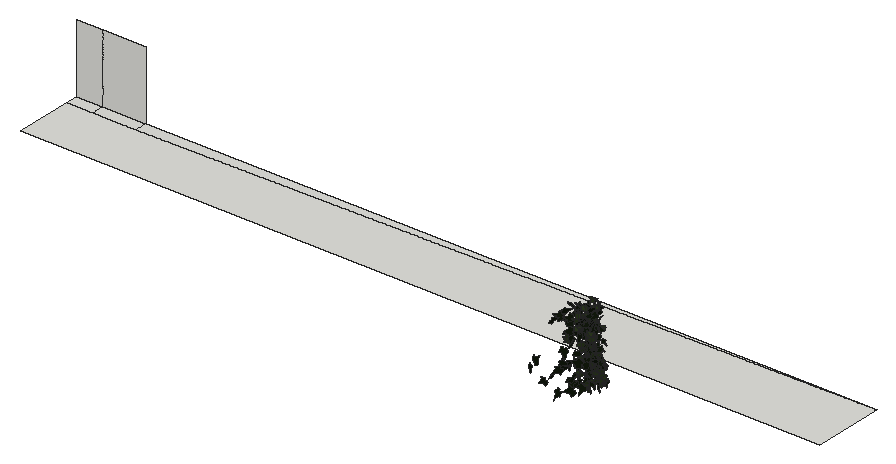
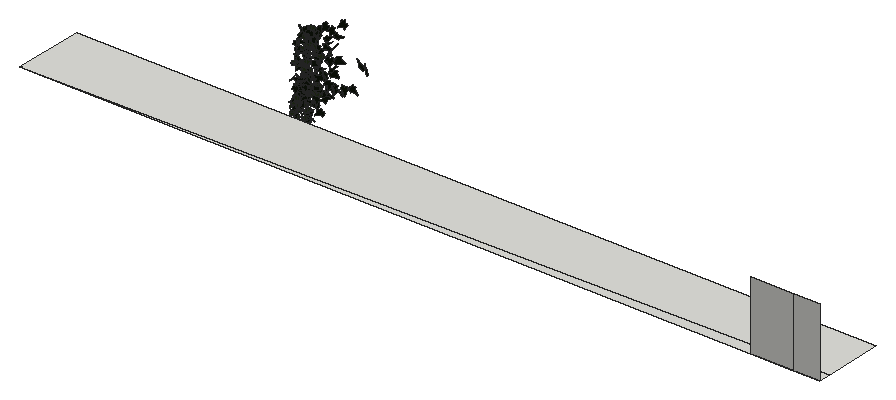
# SketchUp Ruby script. Lengths in inches.
U = 1.inch
M = Sketchup.active_model
def pt(a) = Geom::Point3d.new(a.map { |v| v * U })
def face(e, loops, mat)
  f = e.add_face(loops[0].map { |a| pt(a) })
  loops[1..].each { |l| e.add_face(l.map { |a| pt(a) }).erase! }
  f.material = f.back_material = mat if mat
  f
end
# faces: each face lists its corners as indices into pts; further lists are holes
def faces(e, pts, list, mat = nil) = list.each { |f| face(e, (f[0].is_a?(Array) ? f : [f]).map { |l| l.map { |i| pts[i] } }, mat) }
# xy, xz, yz: faces in a plane at the given z, y or x. An outline is a flat list of corners, or four numbers for a rectangle; further outlines are holes
def ring(l) = l.size == 4 ? [[l[0], l[1]], [l[2], l[1]], [l[2], l[3]], [l[0], l[3]]] : l.each_slice(2).to_a
def flat(e, list, mat, &to3) = list.each { |f| face(e, (f[0].is_a?(Array) ? f : [f]).map { |l| ring(l).map { |u, v| to3.(u, v) } }, mat) }
def xy(e, z, list, mat = nil) = flat(e, list, mat) { |x, y| [x, y, z] }
def xz(e, y, list, mat = nil) = flat(e, list, mat) { |x, z| [x, y, z] }
def yz(e, x, list, mat = nil) = flat(e, list, mat) { |y, z| [x, y, z] }
def lines(e, pts, list) = list.each { |a, b| e.add_line(pt(pts[a]), pt(pts[b])) }
# prism: a flat outline (further loops are holes) pulled along v
def prism(e, loops, v, mat = nil)
  f = face(e, loops, mat); d = Geom::Vector3d.new(v.map { |x| x * U })
  f.pushpull(f.normal.samedirection?(d) ? d.length : -d.length)
end
def box(e, o, s, mat = nil) = prism(e, [[o, [o[0] + s[0], o[1], o[2]], [o[0] + s[0], o[1] + s[1], o[2]], [o[0], o[1] + s[1], o[2]]]], [0, 0, s[2]], mat)
def at(x, y, z, deg = 0) = Geom::Transformation.translation(pt([x, y, z])) * Geom::Transformation.rotation(ORIGIN, Z_AXIS, deg.degrees)
def axes(o, x, y, z) = Geom::Transformation.new([*x, 0, *y, 0, *z, 0, *pt(o).to_a, 1])
def part(name) = M.definitions.add(name)
# library, detail: a bought-in or finely detailed component or shape, given as its bounding box
def library(name, o, s) = part(name).tap { |d| box(d.entities, o, s) }
def detail(e, o, s) = box(e.add_group.entities, o, s)
def put(e, d, t, mat = nil) = e.add_instance(d, t).tap { |i| i.material = mat if mat }
def group(e, t, mat = nil) = e.add_group.tap { |g| g.transformation = t; g.material = mat if mat }.entities
root = M.entities
M.materials.add("efeu1").color = [18, 25, 13]
M.materials.add("efeu2").color = [43, 57, 29]
c1 = part("ivyleaf_9")
p = [[1.54,2.16,1.25],[1.36,2.04,1.19],[-0.21,0.99,0.68],[-0.71,1.11,0.82],[-0.85,0.86,0.67],[-0.8,0.17,0.21],
  [-0.9,-0.01,0.1],[-0.67,-0.16,-0.02],[-0.08,-0.08,-0.05],[-0.03,-0.6,-0.4],[0.65,-0.88,-0.66],[0.83,-0.6,-0.49],
  [1.29,-0.42,-0.43],[1.8125,-0.07,-0.26],[1.21,0.44,0.15]]
faces(c1.entities,p,[[0,1,2,3,4,5,6,7,8,9,10,11,12,13,14]],"efeu1")
c2 = part("ivyleaf_10")
p = [[0,0.5,-0.03],[-0.0625,2.02,-0.43],[-0.19,2.01,-0.46],[-0.54,1.05,-0.29],[-0.52,0.625,-0.18],[-0.83,0.76,-0.28],
  [-1.16,0.64,-0.33],[-1.15,0.33,-0.24],[-0.77,-0.39,0.02],[-0.3,-0.51,0.16],[0.04,-0.48,0.23],[-0.02,2.01,-0.4375],
  [-0.06,2.01,-0.43],[0.04,-0.49,0.23],[0.67,-0.49,0.14],[1.38,0.36,-0.2],[1.375,0.51,-0.24],[0.81,0.65,-0.19],
  [0.62,0.59,-0.15],[0.6,1.09,-0.28],[0.5,1.23,-0.31]]
faces(c2.entities,p,[[0,1,2,3,4,5,6,7,8,9,10],[11,12,0,13,14,15,16,17,18,19,20]],"efeu2")
xy(root,212.04,[[222.91,139.625,222.91,166.9375,255.63,166.9375,600,172.6875,600,139.625],[222.91,166.9375,235.22,172.6875],[235.22,166.9375,255.63,172.6875],[255.63,166.9375,255.63,172.6875,600,172.6875]])
xz(root,172.6875,[[222.91,212.04,235.22,244.35],[235.22,212.04,255.63,244.35]])
put(root,c1,axes([489.04,107.25,219.34],[-0.10171,0.33302,1.23895],[0.37987,-1.13822,0.35983],[1.28078,0.36403,-0.00833]))
put(root,c1,axes([490.16,108.75,221.96],[-0.5052,0.59256,1.08878],[0.68053,-0.83616,0.78501],[1.10672,0.78465,0.01431]))
put(root,c1,axes([491.3,122.97,236.84],[0.60854,-1.02373,-0.20138],[-0.03753,0.20155,-1.21337],[1.12461,0.56068,0.06847]))
put(root,c1,axes([492.44,122.89,218.13],[0.00554,0.22522,1.15832],[-0.28561,1.08343,-0.22658],[-1.19352,-0.25822,0.0596]))
put(root,c1,axes([492.76,111.33,214.01],[0.17278,0.17118,-1.1899],[-1.04476,-0.61365,-0.23616],[-0.68521,0.97881,0.06004]))
put(root,c1,axes([493.82,114.29,214.9],[-0.08217,1.18063,0.10076],[-0.01963,0.09591,-1.23034],[-1.27922,-0.0773,0.01241]))
put(root,c1,axes([494.79,118.48,238.45],[-0.64696,-0.31659,-0.96088],[-0.78751,-0.5761,0.69698],[-0.70174,0.9384,0.10371]))
put(root,c1,axes([494.4,122.13,230.3],[0.37874,1.0301,-0.29598],[-0.09362,-0.27112,-1.13167],[-1.15038,0.3612,-0.00535]))
put(root,c1,axes([494.75,127.88,235.37],[-0.39311,-0.35611,0.92517],[-0.58208,-0.71072,-0.52523],[0.85566,-0.64709,0.06774]))
put(root,c1,axes([494.61,135.09,209.74],[-0.35512,-0.73439,0.18051],[-0.06081,-0.17104,-0.81552],[0.7538,-0.35977,0.01925]))
put(root,c1,axes([495.09,134.37,208.07],[-0.2856,0.78411,0.05143],[-0.00592,0.05257,-0.83441],[-0.78577,-0.28539,-0.0124]))
put(root,c2,axes([494.82,134.58,209.49],[-0.74125,-0.3012,-0.23294],[0.22767,0.05803,-0.79952],[0.30521,-0.77482,0.03067]))
put(root,c2,axes([495.11,126.38,233.46],[-1.07293,-0.21408,0.10536],[-0.11451,0.01138,-1.05635],[0.22873,-0.99855,-0.03462]))
put(root,c1,axes([495.25,134.47,212.06],[-0.74459,-0.40023,0.0405],[0.06147,-0.19741,-0.82066],[0.39755,-0.71908,0.20275]))
put(root,c1,axes([494.92,134.7,208.4],[-0.01052,-0.81612,-0.20319],[-0.01922,0.20338,-0.81591],[0.84081,-0.00556,-0.02119]))
put(root,c1,axes([494.39,118.89,216.28],[0.4027,0.73789,-0.93408],[0.35266,0.83876,0.85764],[1.20483,-0.49214,0.06117]))
put(root,c1,axes([495.07,123.52,223.59],[-0.43715,1.00274,0.10617],[0.02617,-0.1003,1.1245],[1.08825,0.40522,0.0156]))
put(root,c1,axes([495.72,128.53,216.39],[-0.01838,1.02527,0.09743],[-0.1177,0.09137,-1.06061],[-1.10566,-0.02677,0.11129]))
put(root,c2,axes([495.24,134.92,208.11],[0.52925,0.64171,-0.07514],[-0.05706,-0.05033,-0.83172],[-0.64357,0.53218,0.01194]))
put(root,c1,axes([495.95,133.42,216.8125],[-0.78489,-0.15812,0.33707],[-0.31655,-0.13059,-0.79838],[0.19599,-0.84417,0.06037]))
put(root,c2,axes([495.66,135,209.41],[0.3353,-0.66129,-0.38228],[-0.04268,0.40061,-0.73044],[0.76263,0.31316,0.1272]))
put(root,c2,axes([495.7,134.72,210.81],[0.07658,-0.84372,-0.04713],[0.00665,0.04792,-0.84712],[0.84501,0.07609,0.01093]))
put(root,c2,axes([495.69,133.97,213.78],[0.35332,0.70703,-0.3529],[-0.21969,-0.28344,-0.78782],[-0.75905,0.41114,0.06375]))
put(root,c2,axes([496.22,120.92,227.69],[0.43574,0.65548,0.79497],[-0.4783,-0.62404,0.79963],[0.97668,-0.59804,0.03693]))
put(root,c1,axes([495.8125,111.77,240.32],[-0.17706,0.50903,-1.10678],[-0.31093,1.02469,0.55585],[1.23554,0.33081,-0.01872]))
put(root,c1,axes([495.32,119.21,240.76],[0.36831,0.76242,-0.76182],[0.21461,0.70974,0.86447],[1.12152,-0.38619,0.08475]))
put(root,c1,axes([495.51,119.29,224.43],[0.02529,-1.31148,-0.08317],[0.02017,0.08031,-1.364],[1.41888,0.02224,0.02088]))
put(root,c1,axes([495.9,120.45,218.71],[1.00104,0.79642,-0.22113],[-0.17622,-0.13636,-1.27093],[-0.87265,0.94114,0.00298]))
put(root,c1,axes([496.11,134.12,218.96],[-0.67862,-0.51522,-0.21541],[0.17418,0.12681,-0.85204],[0.53058,-0.70061,0.00419]))
put(root,c1,axes([496.35,121.51,215.83],[-0.00738,-0.02583,1.12303],[0.13343,1.07275,0.0275],[-1.1589,0.12368,-0.00399]))
put(root,c2,axes([495.9,128.08,217.55],[0.55185,0.78022,0.48086],[0.16955,0.4466,-0.96419],[-0.9647,0.52481,0.10562]))
put(root,c1,axes([495.68,122.23,235.11],[-0.42552,-0.38668,-1.13477],[0.95435,0.6441,-0.56924],[0.80764,-0.96484,0.07477]))
put(root,c2,axes([496.41,134.01,216.16],[0.10607,-0.86802,0.02616],[0.03421,-0.02215,-0.87392],[0.86774,0.10697,0.03125]))
put(root,c1,axes([496.66,134,223.16],[0.03161,0.8889,-0.11605],[-0.0938,-0.11221,-0.885],[-0.89153,0.04333,0.08899]))
put(root,c1,axes([497.13,121.32,237.29],[-0.34227,-0.13974,1.01438],[-0.9724,-0.37511,-0.36014],[0.43225,-0.9545,-0.00698]))
put(root,c1,axes([496.23,134.41,219.35],[0.81492,0.33541,0.00747],[0.00913,-0.00256,-0.88122],[-0.33537,0.81495,-0.00584]))
put(root,c1,axes([496.87,132.89,222],[-0.8299,-0.28092,-0.1811],[0.16449,0.07871,-0.8759],[0.29096,-0.84578,-0.02136]))
put(root,c2,axes([496.56,127.25,240.54],[-0.52467,0.90112,-0.27806],[0.09577,-0.25568,-1.06379],[-1.01061,-0.49205,0.04355]))
put(root,c2,axes([496.87,119.94,230.12],[0.1837,0.49778,-1.0049],[-0.27761,-0.93184,-0.54632],[-1.14059,0.30697,-0.02888]))
put(root,c1,axes([496.47,134.1875,216.04],[0.82755,0.25066,0.12672],[0.11325,0.06301,-0.86426],[-0.25703,0.83482,0.02718]))
put(root,c1,axes([497.01,132.18,223.83],[0.6338,0.33055,-0.55532],[-0.56454,-0.09539,-0.7011],[-0.31455,0.83724,0.13936]))
put(root,c2,axes([496.85,133.9,222.86],[-0.28737,-0.74179,-0.41221],[0.19652,0.36521,-0.7942],[0.82556,-0.34514,0.04557]))
put(root,c1,axes([496.72,131.95,219.43],[-0.59525,-0.24803,-0.60884],[0.63437,-0.00111,-0.61976],[0.17257,-0.85148,0.17816]))
put(root,c1,axes([497.27,130.99,224.3125],[-0.70407,0.42179,-0.39466],[0.28516,-0.28731,-0.81579],[-0.50234,-0.75427,0.09004]))
put(root,c1,axes([496.58,121.4375,243.24],[1.26723,-0.02604,-0.14385],[-0.1492,0.00917,-1.22058],[0.02908,1.18145,0.0063]))
put(root,c1,axes([497.53,116.6,220.98],[0.0176,0.40263,-1.05478],[-0.18674,-1.00056,-0.41599],[-1.16362,0.16666,0.05081]))
put(root,c2,axes([497.49,133.57,222.47],[-0.28073,0.77431,0.37785],[-0.48797,0.18463,-0.7409],[-0.71008,-0.433,0.35977]))
put(root,c1,axes([497.18,134.35,212.86],[-0.38053,-0.65159,0.39941],[0.01313,-0.45169,-0.72437],[0.76415,-0.31672,0.21134]))
put(root,c2,axes([497.77,124.78,228.36],[-0.49792,0.36679,0.90054],[-0.69462,0.58056,-0.6119],[-0.74093,-0.79076,-0.03153]))
put(root,c1,axes([496.55,124.66,208.33],[-0.12706,-0.23054,-1.1665],[0.80548,0.84016,-0.26095],[0.93841,-0.75236,0.06604]))
put(root,c2,axes([497.17,130.19,222.05],[0.03241,0.77652,0.47703],[0.03444,0.47594,-0.7771],[-0.91069,0.04563,-0.01241]))
put(root,c1,axes([496.93,121.52,230.01],[0.03418,-1.08707,0.40155],[0.00759,-0.38606,-1.13102],[1.24587,0.03217,-0.00413]))
put(root,c2,axes([497.3,129.8125,227.94],[-0.66296,0.75601,-0.01249],[0.01752,-0.00229,-1.01273],[-0.8164,-0.61397,-0.0116]))
put(root,c1,axes([498.02,129.76,207.95],[-1.02692,0.09772,-0.02308],[0.01806,-0.05412,-0.99262],[-0.10671,-0.94957,0.0542]))
put(root,c1,axes([498.33,129.82,217.5625],[-0.68141,0.55611,0.37114],[-0.47007,0.02148,-0.83511],[-0.53694,-0.72455,0.26011]))
put(root,c1,axes([497.4,134.97,208.01],[0.12814,-0.82287,0.0192],[-0.01266,-0.0214,-0.83264],[0.82299,0.1278,-0.0158]))
put(root,c1,axes([497.09,124.03,229.93],[0.17337,0.05719,1.19004],[1.09141,0.53733,-0.17537],[-0.58299,1.02294,0.02558]))
put(root,c2,axes([498.13,129.73,217.26],[-0.66019,-0.61668,0.06954],[-0.04787,-0.05063,-0.90339],[0.61874,-0.66191,0.00431]))
put(root,c1,axes([498.33,124.97,240.39],[-0.17221,-0.17296,0.99814],[-0.73804,-0.67397,-0.2444],[0.75138,-0.70164,-0.0113]))
put(root,c2,axes([498.1,132.97,227.38],[0.4241,-0.81769,-0.1481],[0.01828,0.17541,-0.91614],[0.8308,0.41356,0.09576]))
put(root,c1,axes([497.87,120.74,211.82],[-0.44173,-1.07457,-0.32087],[0.08631,0.29958,-1.19534],[1.20434,-0.4156,-0.03202]))
put(root,c1,axes([497.61,129.2,209.98],[1.05315,0.04965,0.01164],[0.0104,0.03101,-1.01496],[-0.05398,0.97471,0.0317]))
put(root,c2,axes([498.61,126.66,236.45],[0.77714,-0.37747,-0.70181],[-0.62806,0.34334,-0.84463],[0.55036,0.92482,0.02712]))
put(root,c1,axes([498.61,132.15,234.54],[-0.94064,-0.1192,-0.01452],[0.0258,-0.08869,-0.94377],[0.11727,-0.93656,0.09122]))
put(root,c1,axes([499.03,130.09,234.77],[-0.73853,0.4433,0.41509],[-0.3527,0.21893,-0.86134],[-0.49439,-0.8184,-0.00558]))
put(root,c1,axes([497.59,123.98,242.3125],[1.19558,-0.32993,0.12373],[0.14956,0.04925,-1.19798],[0.34801,1.1123,0.08975]))
put(root,c2,axes([498.48,133.2,227.78],[0.14103,-0.68346,-0.59855],[0.015,0.60739,-0.69002],[0.90838,0.09608,0.10432]))
put(root,c1,axes([499.19,126.16,228.85],[-0.13747,-0.04116,-1.01678],[-0.77798,-0.66334,0.12658],[-0.71528,0.7294,0.05774]))
put(root,c1,axes([498.89,119.32,233.1],[-0.37167,-0.2722,1.10926],[-0.7985,-0.77075,-0.45266],[0.88076,-0.81363,0.05771]))
put(root,c1,axes([499.12,123.29,240.79],[-0.1657,0.99448,0.58892],[-0.33728,0.51327,-1.02545],[-1.18904,-0.28418,0.20881]))
put(root,c1,axes([498.4,129.68,217.16],[0.08554,-0.13683,-0.93531],[-0.31118,0.85248,-0.16128],[0.93187,0.29723,0.032]))
put(root,c1,axes([498.97,130.38,209.625],[-0.11439,-0.78391,-0.54757],[-0.0898,-0.52001,0.8226],[-1.0159,0.13424,-0.01106]))
put(root,c1,axes([498.09,123.8125,220.88],[-0.30373,-0.18235,1.16396],[1.16529,0.31165,0.33477],[-0.3767,1.1111,0.09712]))
put(root,c1,axes([498.4,129.6875,225.82],[-0.16275,-0.92079,0.03748],[-0.00431,-0.0373,-0.93506],[0.92155,-0.16279,0.00225]))
put(root,c1,axes([499.3,124.7,224.89],[-0.63767,0.25231,-0.72477],[-0.70711,0.24001,0.66728],[0.37513,0.88129,0.02578]))
put(root,c1,axes([499.5625,127.11,224.41],[-0.69135,0.61207,0.60328],[-0.48856,0.36537,-0.92012],[-0.7686,-0.78279,0.04223]))
put(root,c1,axes([499.15,111.75,211.05],[-1.31922,0.09386,-0.42953],[0.44102,-0.07361,-1.27343],[-0.1214,-1.28733,0.04149]))
put(root,c2,axes([498.31,123.35,232.8],[0.69691,0.48531,0.5784],[0.48562,0.32737,-0.83968],[-0.63219,0.78646,-0.00739]))
put(root,c1,axes([498.31,130.29,207.71],[0.98175,-0.29555,-0.03879],[-0.03963,0.00775,-0.9941],[0.31927,0.90976,-0.00413]))
put(root,c1,axes([498.77,123.82,234.75],[0.65604,0.73331,0.15794],[0.08164,0.13449,-0.9899],[-0.80464,0.61152,0.02833]))
put(root,c2,axes([498.38,132.61,229.54],[0.73165,0.15383,0.57334],[0.54485,0.1872,-0.74551],[-0.23564,0.91049,0.05641]))
put(root,c1,axes([498.29,132.42,225.6875],[0.81378,0.08466,0.41578],[0.41416,0.03703,-0.81815],[-0.09225,0.91309,-0.00537]))
put(root,c1,axes([497.98,122.87,216.52],[1.07921,-0.48847,0.50036],[0.46667,-0.21156,-1.15676],[0.57491,1.08869,-0.00029]))
put(root,c1,axes([499.36,123.89,224.65],[0.15653,-0.90706,0.60586],[-0.10099,0.57501,0.95531],[-1.15988,-0.17248,-0.00141]))
put(root,c2,axes([498.44,123.09,218.04],[-0.60621,0.16778,-0.87248],[0.8574,-0.27182,-0.60896],[-0.34438,-0.97209,0.01969]))
put(root,c1,axes([498.65,129.76,239.6],[-0.02126,0.17413,0.96713],[0.2079,-0.90994,0.18144],[1.00041,0.1928,-0.01716]))
put(root,c1,axes([499.57,124.65,217.37],[-0.85023,-0.42758,0.44075],[-0.397,-0.21111,-0.93166],[0.51491,-0.8688,0.00946]))
put(root,c2,axes([498.71,122.86,213.92],[0.25345,0.54074,0.79376],[0.31051,0.70709,-0.61294],[-0.9613,0.37097,0.01129]))
put(root,c1,axes([498.53,124.3,209.86],[-0.08457,0.11147,1.02734],[0.5133,-0.8661,0.14082],[0.94297,0.48146,0.01548]))
put(root,c1,axes([499.43,126.4375,234.16],[-0.91658,0.28737,-0.32972],[0.31554,-0.12533,-0.93154],[-0.33764,-0.89726,0.02452]))
put(root,c2,axes([498.6875,129.87,224.97],[-0.03678,0.0072,-0.99469],[0.77939,0.62828,-0.02181],[0.67793,-0.72193,-0.0289]))
put(root,c2,axes([499.7,130.89,242.03],[-0.86623,0.10035,0.44623],[-0.45699,-0.15074,-0.85322],[-0.01874,-0.96268,0.18012]))
put(root,c1,axes([498.98,131.43,235.375],[-0.37926,-0.79752,-0.36037],[0.43282,0.17043,-0.83269],[0.76064,-0.49463,0.29413]))
put(root,c2,axes([499.33,130.51,238.68],[-0.32152,0.82464,-0.3916],[-0.10297,-0.44529,-0.85315],[-0.90707,-0.24175,0.23566]))
put(root,c2,axes([499.96,131,215.89],[-0.06646,0.03335,0.96104],[-0.87996,0.43597,-0.07279],[-0.47222,-0.8171,0.00039]))
put(root,c1,axes([499.8,124.54,233.64],[-0.92479,0.61939,-0.34605],[0.27773,-0.21212,-1.09889],[-0.70674,-0.89384,0.02098]))
put(root,c1,axes([498.875,129.97,223.84],[0.50252,-0.83473,-0.05917],[-0.02961,0.04985,-0.99388],[0.90311,0.4661,0.00033]))
put(root,c1,axes([499.74,132.2,236.03],[-0.90783,-0.27021,-0.19313],[0.22187,-0.07509,-0.93788],[0.24716,-0.92511,0.13254]))
put(root,c2,axes([499.2,124.12,220.125],[-0.90232,-0.07225,-0.58232],[0.60577,0.00764,-0.87144],[0.06942,-1.00573,0.03521]))
put(root,c2,axes([499.66,125.43,223.32],[-0.07199,-0.9255,-0.07265],[0.01646,0.06894,-0.96495],[1.00225,-0.0676,0.01062]))
put(root,c2,axes([499.49,129.3,230.98],[0.70318,0.75871,0.0404],[0.02931,0.0279,-1.03977],[-0.81995,0.65166,-0.00252]))
put(root,c2,axes([499.82,134.2,214.39],[-0.0503,-0.85595,-0.12657],[0.01219,0.12607,-0.85742],[0.86517,-0.05154,0.00473]))
put(root,c2,axes([499.85,128.72,233.84],[0.71613,-0.71314,-0.30994],[-0.10482,0.31273,-1.00286],[0.82813,0.65628,0.14108]))
put(root,c2,axes([499.95,134.36,214.45],[-0.40499,-0.74938,0.15285],[-0.01894,-0.16308,-0.8497],[0.76457,-0.40098,0.05992]))
put(root,c1,axes([499.93,131.25,218.58],[0.34181,0.85227,0.09917],[0.05588,0.08248,-0.94528],[-0.92451,0.32008,-0.02047]))
put(root,c1,axes([499.32,123.07,239.6875],[1.02219,-0.59304,-0.23328],[-0.19368,0.13617,-1.16141],[0.6568,0.96311,0.02057]))
put(root,c1,axes([500.04,126.3,223.77],[0.39361,-0.25395,-0.97233],[-0.82974,0.53277,-0.46197],[0.63742,0.85033,-0.00094]))
put(root,c2,axes([499.13,130.65,206.77],[0.36879,-0.05761,-0.91913],[0.95424,-0.04302,0.35796],[-0.06582,-0.94648,0.03967]))
put(root,c2,axes([500.18,127.18,227.8],[-0.22906,0.76849,-0.55779],[-0.13167,0.5226,0.8289],[1.00351,0.24399,-0.01856]))
put(root,c2,axes([500,125.29,233.5625],[0.73235,-0.86183,-0.05062],[-0.03016,0.03995,-1.14048],[0.93177,0.67867,0.00287]))
put(root,c1,axes([500.54,128.22,234.75],[-1.10687,0.01128,0.1043],[-0.10892,-0.07671,-1.0629],[-0.00402,-1.02692,0.08054]))
put(root,c1,axes([500.25,124.22,240.49],[-0.84758,0.38507,-0.43315],[0.38508,-0.21808,-0.90842],[-0.47644,-0.86129,0.03636]))
put(root,c1,axes([499.29,129.29,226.3],[0.89534,-0.08112,0.40909],[0.42318,-0.03468,-0.86629],[0.09521,0.91695,0.00343]))
put(root,c2,axes([500,127.57,240.4],[0.79665,-0.58142,0.10459],[0.08195,-0.06513,-0.98625],[0.58504,0.80084,-0.00427]))
put(root,c2,axes([500.64,121.92,216.85],[0.29042,0.1278,-1.06263],[-0.61613,0.89763,-0.03938],[0.92582,0.55728,0.30712]))
put(root,c2,axes([500.31,127.6875,237.49],[0.90473,0.43672,-0.47132],[-0.46007,-0.16194,-0.98123],[-0.50035,0.93857,0.05]))
put(root,c1,axes([500.22,132.2,213.98],[-0.65736,-0.56371,0.30057],[0.00351,-0.40358,-0.81153],[0.68415,-0.53956,0.29297]))
put(root,c1,axes([499.77,134.38,213.53],[0.18804,-0.83335,0.10377],[0.02658,-0.10038,-0.85429],[0.83937,0.18987,0.0038]))
put(root,c2,axes([500.24,131.89,206.17],[0.34971,-0.768,-0.16209],[-0.04525,0.15743,-0.84355],[0.78362,0.35183,0.02362]))
put(root,c1,axes([499.79,127.06,230.91],[0.00482,-1.05742,-0.21449],[0.06454,0.20616,-1.09798],[1.16174,-0.00706,0.06189]))
put(root,c2,axes([500.48,134.13,217.45],[-0.83334,-0.16244,0.23055],[-0.22327,-0.05944,-0.84889],[0.17232,-0.8626,0.01508]))
put(root,c1,axes([500.22,126.62,241.625],[0.95183,0.51386,-0.41668],[-0.41265,-0.13836,-1.05864],[-0.57004,0.95818,0.0706]))
put(root,c1,axes([501.03,126.5625,218.49],[-0.11909,0.13228,1.03811],[-1.08526,0.04933,-0.12224],[-0.06908,-1.00304,0.13089]))
put(root,c1,axes([499.875,120.2,221.66],[1.02073,-0.44715,-0.33369],[-0.30803,0.14737,-1.08732],[0.50834,0.98716,0.01118]))
put(root,c1,axes([500.74,127.13,217.28],[-0.90946,-0.36324,0.22394],[0.21293,0.08658,0.95378],[-0.40329,0.86487,-0.00143]))
put(root,c1,axes([499.94,132.99,229.65],[0.11086,-0.7358,-0.55565],[0.19262,0.56579,-0.7108],[0.90169,-0.0304,0.22016]))
put(root,c2,axes([500.59,123.18,226.77],[-0.7352,-0.8394,-0.00642],[0.00081,0.00734,-1.12396],[0.90657,-0.68073,-0.0042]))
put(root,c1,axes([500.38,131.3,226.98],[-0.72438,0.01747,-0.59204],[0.60661,-0.12536,-0.69224],[-0.10187,-0.87076,0.08778]))
put(root,c1,axes([500.18,123.42,237.36],[0.96949,0.66828,0.08804],[0.06339,0.06291,-1.16377],[-0.72474,0.89946,0.01599]))
put(root,c2,axes([500.23,126.6,229.84],[-0.81521,0.49077,-0.41504],[0.33017,-0.2609,-0.93505],[-0.59807,-0.81299,0.04952]))
put(root,c2,axes([500.28,125.84,235.4],[0.1232,0.97799,0.3591],[0.05441,0.34174,-1.02395],[-1.1188,0.12431,-0.01025]))
put(root,c2,axes([500.61,126.45,240.15],[-1.0373,-0.50003,-0.02992],[0.03191,0.00553,-1.1261],[0.53998,-0.96088,0.00908]))
put(root,c1,axes([501.2,127.39,214.9],[-0.42348,-0.43714,-0.68184],[-0.47872,-0.48309,0.6107],[-0.70361,0.59178,-0.00513]))
put(root,c2,axes([500.46,122.3,219.9375],[-1.10661,0.21848,-0.1847],[0.19035,-0.02497,-1.0895],[-0.23713,-1.03961,-0.01265]))
put(root,c2,axes([501.0625,127.57,224.48],[-0.95947,-0.0351,0.55145],[-0.57126,-0.04074,-0.92448],[0.05509,-1.0338,0.01771]))
put(root,c1,axes([501.09,109.86,222.25],[-0.16495,0.06879,-1.34198],[-0.07788,-1.29778,-0.06308],[-1.3934,0.06439,0.16239]))
put(root,c1,axes([501.3,128.23,226.96],[-0.48672,0.61917,0.55677],[-0.33589,0.43577,-0.79644],[-0.81771,-0.54755,-0.00425]))
put(root,c2,axes([500.96,129.78,223.26],[0.1073,-0.04662,-0.96659],[-0.27998,0.89631,-0.07558],[0.96524,0.26516,0.08553]))
put(root,c2,axes([500.41,126.34,221.6],[-0.03099,-0.2925,-0.90066],[0.27162,-0.83553,0.28483],[-0.94911,-0.22956,0.11092]))
put(root,c1,axes([501.7,116.54,210.55],[-0.26535,-0.1554,-1.33294],[-0.8372,-1.02556,0.28387],[-1.11503,0.80701,0.10406]))
put(root,c1,axes([501.11,132.09,219.73],[-0.01644,0.19408,-0.85097],[-0.13778,-0.80944,-0.1972],[-0.89771,0.12068,0.04585]))
put(root,c2,axes([500.72,125.92,222.78],[-0.06477,0.74956,0.74363],[-0.10384,0.70911,-0.78147],[-1.11395,-0.10969,0.02961]))
put(root,c1,axes([500.48,126.78,218.94],[0.07833,0.4036,-0.82541],[0.05053,0.79347,0.42408],[0.9603,-0.07467,0.04502]))
put(root,c2,axes([500.72,126.43,224.0625],[-0.00898,0.31388,-0.87062],[0.00354,-0.83716,-0.32647],[-0.96556,-0.00599,0.0069]))
put(root,c1,axes([501.39,127.68,237.18],[-0.09006,-0.06986,-1.0053],[-0.33642,-0.9168,0.09686],[-0.99115,0.31753,0.05847]))
put(root,c1,axes([501.68,125.23,216.78],[-0.20404,0.03206,1.03357],[-1.07156,0.06039,-0.19818],[-0.07056,-1.00981,0.02097]))
put(root,c1,axes([500.52,132.64,231.51],[0.21833,-0.91678,-0.02062],[-0.00221,0.02067,-0.94241],[0.91701,0.21832,0.00263]))
put(root,c1,axes([501.29,125.91,236.4],[0.41034,-0.0779,-0.95814],[-0.98447,0.13505,-0.40284],[0.16703,0.98737,-0.02049]))
put(root,c2,axes([501.1,122.58,214.65],[-0.19101,-0.9346,0.42419],[-0.03944,-0.40789,-0.9885],[1.1006,-0.17682,0.03819]))
put(root,c1,axes([501.7,125.24,235.02],[-1.17464,0.07906,0.29967],[-0.31322,-0.01765,-1.13345],[-0.07763,-1.12501,0.03885]))
put(root,c1,axes([500.32,128.9,224.71],[0.67119,-0.73828,0.24572],[0.18848,-0.16179,-1.0032],[0.81568,0.64489,0.02962]))
put(root,c1,axes([501.53,131.75,216.58],[-0.6096,0.69623,0.10403],[-0.05269,0.0892,-0.93195],[-0.75782,-0.56626,-0.01889]))
put(root,c1,axes([500.98,126.9,224.11],[-0.5552,-0.89143,0.00533],[-0.00254,-0.00456,-1.0702],[0.96275,-0.51408,0.00025]))
put(root,c1,axes([501.39,132.51,233.31],[-0.12939,0.76527,0.37778],[-0.02808,0.36337,-0.80506],[-0.91444,-0.11944,-0.02873]))
put(root,c1,axes([500.5625,131.44,242.35],[0.82139,-0.55445,-0.03092],[0.00973,0.06957,-0.989],[0.55522,0.81903,0.06307]))
put(root,c1,axes([501.55,132.84,225.84],[-0.84608,0.21227,-0.16344],[0.16316,-0.04335,-0.84412],[-0.23396,-0.79784,0.00238]))
put(root,c1,axes([501.93,131.01,219.39],[-0.35901,-0.03329,0.86529],[-0.89591,-0.06435,-0.34737],[0.07788,-0.89364,-0.00723]))
put(root,c2,axes([501.02,129.81,224.08],[-0.63963,0.60377,-0.41437],[0.2962,-0.28908,-0.87956],[-0.72293,-0.65264,0.00625]))
put(root,c1,axes([500.95,131.08,217.0625],[0.50697,0.66282,0.27932],[-0.16378,-0.2217,0.84468],[0.75481,-0.49329,-0.00432]))
put(root,c2,axes([501.15,120.39,240.46],[0.14546,1.03327,0.1315],[0.02164,0.1249,-1.08368],[-1.12405,0.13612,-0.00385]))
put(root,c1,axes([501.53,123.02,209.17],[-1.11925,-0.55974,-0.26277],[0.25562,0.09328,-1.22457],[0.61201,-1.06261,0.03091]))
put(root,c2,axes([501.6,131.99,239.52],[-0.56104,0.61003,0.33231],[-0.20214,0.26011,-0.83292],[-0.71575,-0.55164,-0.02525]))
put(root,c1,axes([501.76,132.76,216.75],[-0.27236,0.68464,-0.38635],[0.14228,-0.34736,-0.75878],[-0.82912,-0.2845,-0.0033]))
put(root,c2,axes([501.67,131.69,239.58],[-0.00304,0.36673,0.82898],[-0.3702,0.73329,-0.35213],[-0.87229,-0.31249,0.14655]))
put(root,c1,axes([501.3,127.65,224.02],[-0.40039,-0.93785,-0.24413],[0.14398,0.19942,-1.04755],[1.03415,-0.39086,0.05132]))
put(root,c1,axes([501.74,132.45,233.55],[0.17901,0.58463,0.62517],[-0.0268,0.61591,-0.61585],[-0.90522,0.09738,0.14186]))
put(root,c1,axes([501.8125,126.37,226.24],[0.66459,0.18743,-0.75447],[-0.76212,-0.1706,-0.66836],[-0.27203,0.93587,0.02926]))
put(root,c1,axes([501.56,127.94,222.52],[0.53505,0.87984,0.17678],[0.09381,0.14616,-1.05011],[-0.96324,0.50296,-0.00407]))
put(root,c2,axes([501.71,127.04,234.65],[-0.26443,0.69768,0.56768],[0.03711,-0.55841,0.75831],[0.95598,0.21466,0.12759]))
put(root,c1,axes([502.07,132,236.99],[-0.24447,0.57553,-0.62711],[-0.06411,-0.63437,-0.60653],[-0.89797,-0.1114,0.21404]))
put(root,c2,axes([501.125,126.38,206.85],[-0.22491,0.02697,0.88455],[0.80616,-0.41466,0.20375],[0.44129,0.77125,0.07861]))
put(root,c1,axes([501.76,133.1,220.65],[0.60618,0.41363,-0.41729],[-0.34734,-0.23993,-0.72511],[-0.51642,0.64689,-0.00212]))
put(root,c1,axes([501.25,129.86,219.36],[0.32997,-0.56215,-0.65112],[0.04426,0.70755,-0.58844],[0.85908,0.17946,0.28041]))
put(root,c2,axes([501.74,132.94,229.74],[-0.15143,0.37218,-0.76544],[-0.15418,-0.74624,-0.36417],[-0.87729,0.06691,0.19612]))
put(root,c1,axes([502.43,130.49,223.18],[-0.42319,0.42616,0.652],[-0.51901,0.40615,-0.5995],[-0.63316,-0.61776,0.05564]))
put(root,c2,axes([501.4,123.98,242.3],[0.97887,0.46929,0.29683],[0.22313,0.21898,-1.05679],[-0.54964,0.92466,0.09962]))
put(root,c1,axes([502.49,130.7,220.7],[-0.66049,0.21072,0.56056],[-0.57479,0.10324,-0.67],[-0.2455,-0.80863,0.06054]))
put(root,c1,axes([501.4375,128.4375,208.19],[0.25813,-0.78487,-0.25742],[-0.0733,0.23807,-0.85326],[0.88578,0.24843,0.00441]))
put(root,c1,axes([501.4,128.48,229.04],[-0.1278,0.25264,0.92336],[0.23076,-0.86331,0.2851],[0.96986,0.2387,0.05384]))
put(root,c1,axes([502.02,126.5,234.31],[0.11445,0.5637,0.85194],[0.11399,0.81278,-0.59587],[-1.06786,0.14718,0.0277]))
put(root,c2,axes([501.9375,127.9,233.07],[0.52463,-0.91474,0.13085],[0.06935,-0.10836,-1.07714],[0.99481,0.48996,0.00608]))
put(root,c2,axes([502.47,128.97,234.66],[-0.34903,-0.42252,0.79007],[-0.52259,-0.58587,-0.55296],[0.77992,-0.58165,-0.01694]))
put(root,c2,axes([502.36,130.93,217.48],[-0.81275,0.11365,-0.35016],[-0.35593,0.07169,0.79125],[0.14353,0.82131,-0.02061]))
put(root,c1,axes([502.55,129.69,213.73],[-0.74869,0.65347,-0.04244],[0.01528,-0.04446,-0.99051],[-0.70696,-0.69301,0.02353]))
put(root,c2,axes([502.375,124.52,209.875],[-0.28128,-0.18291,-0.90303],[-0.52859,-0.72522,0.31156],[-0.79938,0.54391,0.11173]))
put(root,c1,axes([502.67,129.57,229.16],[-0.31412,0.598,0.63066],[-0.37021,0.5044,-0.68829],[-0.842,-0.44486,0.06735]))
put(root,c1,axes([501.61,127.53,222.26],[1.00102,0.37828,0.18921],[0.1865,0.05832,-1.04108],[-0.4132,0.94276,-0.01152]))
put(root,c2,axes([502.19,126.67,225.37],[-0.10766,0.33883,0.97783],[-0.28285,0.903,-0.36731],[-1.04164,-0.28023,-0.00132]))
put(root,c1,axes([502.6875,129.86,211.84],[-0.22217,0.90538,0.12654],[-0.36148,0.04135,-0.90849],[-0.91799,-0.2354,0.32711]))
put(root,c2,axes([502.17,133.6,216.31],[0.78776,-0.26887,-0.1863],[-0.17489,0.07849,-0.80828],[0.30193,0.74697,0.01787]))
put(root,c1,axes([502.34,127.86,222.6875],[-0.554,0.61837,-0.33668],[-0.28801,0.19765,0.83209],[0.69663,0.57347,0.07626]))
put(root,c2,axes([502.84,130.14,220.21],[0.05942,0.04999,0.91263],[-0.90161,-0.27212,0.07056],[0.297,-0.83608,0.03161]))
put(root,c2,axes([502.59,128.92,213.08],[-0.91694,-0.07028,0.45333],[-0.44309,-0.22356,-0.86855],[0.17622,-0.92782,0.17494]))
put(root,c1,axes([501.77,126.7,233.37],[0.17289,0.9534,-0.14898],[0.02376,0.14156,1.00541],[1.04096,-0.16158,0.00179]))
put(root,c2,axes([502.4375,127.54,221.22],[-0.20724,-0.88401,0.39362],[-0.09083,-0.36904,-0.94077],[1.03458,-0.20948,-0.00375]))
put(root,c1,axes([502.36,133.87,215.21],[-0.3767,-0.43705,0.55715],[-0.24504,-0.49444,-0.57314],[0.70534,-0.40519,0.09844]))
put(root,c1,axes([502.45,131.72,238.85],[0.28316,0.80297,-0.22237],[-0.07804,-0.20133,-0.87846],[-0.89403,0.2719,0.00625]))
put(root,c2,axes([502.46,126.75,227.96],[-0.98086,-0.58976,0.02152],[0.02715,-0.07661,-1.12329],[0.63676,-0.90521,0.08105]))
put(root,c1,axes([502.65,120.35,237.98],[0.06939,1.14035,0.47251],[0.03959,0.45297,-1.18779],[-1.32513,0.07324,-0.01074]))
put(root,c2,axes([502.03,126.73,217.84],[-0.81244,0.42494,-0.53273],[0.45746,-0.2906,-0.89765],[-0.55443,-0.86245,0.03999]))
put(root,c1,axes([503.17,115.53,216.67],[-1.02472,0.89586,0.09121],[-0.07512,0.05407,-1.35709],[-0.96925,-0.95132,0.00875]))
put(root,c2,axes([502.38,129.32,208.93],[-0.0512,-0.26833,-0.81258],[-0.1279,-0.77233,0.28332],[-0.883,0.12742,0.00608]))
put(root,c2,axes([502.51,135.09,206.46],[0.01569,-0.83075,0.01138],[-0.02778,-0.0119,-0.83043],[0.83036,0.0153,-0.02799]))
put(root,c2,axes([502.89,125.41,230.09],[0.77304,0.25365,0.70201],[-0.67826,-0.24811,0.78955],[0.38272,-0.95206,-0.01872]))
put(root,c1,axes([502.55,135.12,206.09],[-0.03042,0.21163,-0.80134],[-0.48468,0.64594,0.18899],[0.67233,0.47522,0.09999]))
put(root,c1,axes([502.05,132.45,211.99],[-0.0851,-0.22812,-0.80261],[0.26547,0.73155,-0.25099],[0.82759,-0.25812,-0.00202]))
put(root,c2,axes([502.42,128.55,229.05],[-0.63369,0.83576,0.08055],[-0.03538,0.07163,-1.06191],[-0.9058,-0.58749,-0.01488]))
put(root,c1,axes([502.17,131.63,207.74],[0.0191,-0.07635,-0.94329],[-0.05747,0.90554,-0.08036],[0.98135,0.05452,0.01365]))
put(root,c2,axes([503.06,130,210.99],[-0.23472,0.07161,0.79806],[-0.79262,0.22417,-0.23792],[-0.2541,-0.7654,0.00498]))
put(root,c2,axes([502.7,128.51,215.57],[-0.49612,-0.84353,0.05572],[-0.03187,-0.04493,-0.99892],[0.91229,-0.4603,-0.0046]))
put(root,c1,axes([502.79,128.7,237.74],[-0.96743,-0.4036,-0.0786],[0.07503,0.02979,-1.0218],[0.43707,-0.89846,0.00143]))
put(root,c1,axes([502.59,128.34,218.08],[0.6062,0.68579,-0.24521],[-0.17099,-0.17508,-0.92159],[-0.76432,0.58309,0.01168]))
put(root,c1,axes([503.26,128.67,216.375],[-0.61246,0.58222,0.39627],[-0.33725,0.22632,-0.84299],[-0.67156,-0.64464,0.06194]))
put(root,c1,axes([503.04,131.65,216.06],[-0.96175,-0.13577,0.07348],[-0.0561,-0.12429,-0.92921],[0.15549,-0.88462,0.11927]))
put(root,c1,axes([503.0625,131.89,212.99],[0.31167,0.26182,-0.72786],[-0.66115,-0.34738,-0.39767],[-0.46277,0.67262,0.07794]))
put(root,c1,axes([502.94,132.125,213.99],[-0.09456,0.49373,-0.71867],[0.04143,-0.69168,-0.51902],[-0.91629,-0.08222,0.0507]))
put(root,c2,axes([502.28,131.75,208.375],[-0.74963,0.06126,-0.59311],[0.61317,-0.05389,-0.72466],[-0.08806,-0.89672,0.00303]))
put(root,c1,axes([503.78,118.37,221.34],[-0.52209,0.08107,1.20498],[-1.223,0.24606,-0.50928],[-0.27882,-1.23109,-0.02244]))
put(root,c2,axes([502.72,134.98,207.28],[0.15921,-0.77706,0.26102],[0.04989,-0.25622,-0.7932],[0.8182,0.16683,-0.00242]))
put(root,c1,axes([502.375,128.6,241.82],[-0.15182,0.76093,0.6004],[0.12109,-0.56635,0.80474],[1.02443,0.17972,-0.00614]))
put(root,c1,axes([502.82,126.69,231.42],[-0.84561,0.61402,0.12796],[0.08914,-0.09408,1.03455],[0.67043,0.78698,0.02384]))
put(root,c2,axes([502.54,133.45,206.8125],[0.40743,0.64168,0.3781],[0.06385,0.38073,-0.76268],[-0.79395,0.35991,0.1327]))
put(root,c1,axes([502.02,131.46,214.17],[0.5514,-0.42594,0.5652],[0.47943,-0.30224,-0.6955],[0.5206,0.72948,0.04186]))
put(root,c2,axes([502.98,132.36,210.84],[0.06529,0.19242,0.84882],[-0.16157,-0.80269,0.20833],[0.89111,-0.15963,-0.02442]))
put(root,c2,axes([502.73,125.25,207.79],[-0.67511,0.65595,-0.06432],[0.04195,-0.04841,-0.94233],[-0.71033,-0.62628,0.00548]))
put(root,c2,axes([502.88,128.52,215.91],[-0.18851,0.90917,0.29517],[-0.19869,0.25093,-0.95363],[-1.00927,-0.21921,0.13261]))
put(root,c2,axes([503.3,133.03,230.5625],[0.52218,0.12165,-0.66656],[-0.70034,0.00252,-0.50826],[-0.07693,0.80284,0.10259]))
put(root,c1,axes([502.61,135.06,206.72],[0.00903,-0.81708,-0.15844],[0.00636,0.15852,-0.81709],[0.83227,0.00765,0.00797]))
put(root,c2,axes([502.87,128.49,241.04],[0.68504,0.66174,-0.25087],[-0.19535,-0.16069,-0.95311],[-0.73517,0.65932,0.0195]))
put(root,c2,axes([502.68,130.56,220.25],[-0.04741,-0.4429,0.77583],[0.14425,0.73459,0.46175],[-0.9258,0.13714,0.03221]))
put(root,c1,axes([502.66,132.79,230.3],[-0.1468,-0.85586,0.35468],[0.0883,-0.37039,-0.85724],[0.92222,-0.10077,0.13854]))
put(root,c1,axes([502.72,129.25,214.42],[0.54367,-0.62184,-0.48786],[0.31503,-0.36739,0.83205],[-0.78003,-0.58179,-0.00399]))
put(root,c1,axes([503.79,118.48,232.14],[-0.25719,0.64758,1.12534],[-0.50743,0.97633,-0.71522],[-1.26386,-0.52377,0.05815]))
put(root,c2,axes([502.99,134.26,213.58],[-0.27269,0.7087,0.10176],[-0.04624,0.08861,-0.78235],[-0.77127,-0.25588,0.01092]))
put(root,c1,axes([503.45,125.56,241.62],[0.04743,0.89063,-0.5542],[-0.0878,-0.52877,-0.92607],[-1.11746,0.07935,0.04924]))
put(root,c2,axes([503.24,131.21,213.07],[-0.76902,-0.44058,0.01735],[-0.01524,-0.00889,-0.87083],[0.47593,-0.7122,0.00014]))
put(root,c1,axes([502.55,130.65,206.32],[-0.01863,0.00863,-0.88121],[0.9097,-0.09218,-0.01881],[-0.09973,-0.84247,-0.00697]))
put(root,c1,axes([502.58,133.34,224.57],[0.57186,-0.69119,-0.16416],[0.07641,0.26935,-0.86794],[0.7063,0.53049,0.22681]))
put(root,c2,axes([503.58,133.45,209.57],[0.05618,0.32821,-0.815],[-0.72638,-0.44209,-0.2281],[-0.49428,0.68698,0.24259]))
put(root,c2,axes([503.21,130.55,209.51],[-0.9827,-0.1239,-0.03946],[0.05062,-0.06379,-0.9523],[0.13048,-0.90846,0.07225]))
put(root,c2,axes([503.29,131.67,206.35],[-0.05404,0.50178,-0.6637],[-0.08209,0.63368,0.52438],[0.87292,0.09065,0.00822]))
put(root,c2,axes([502.53,133.69,214.28],[0.16596,0.0341,0.79216],[0.76306,0.28572,-0.16154],[-0.30954,0.7226,0.0265]))
put(root,c2,axes([502.6,130.47,233.62],[-0.19616,-0.1525,0.89032],[0.8554,-0.38996,0.10252],[0.38759,0.78344,0.22433]))
put(root,c2,axes([503.3,130.53,220.15],[0.02515,-0.89761,0.29198],[0.01779,-0.2804,-0.93379],[1.01558,0.02714,0.00913]))
put(root,c1,axes([503.83,130.75,222.23],[-0.62577,-0.55518,-0.31617],[-0.23809,-0.20935,0.83456],[-0.64081,0.61993,-0.00132]))
